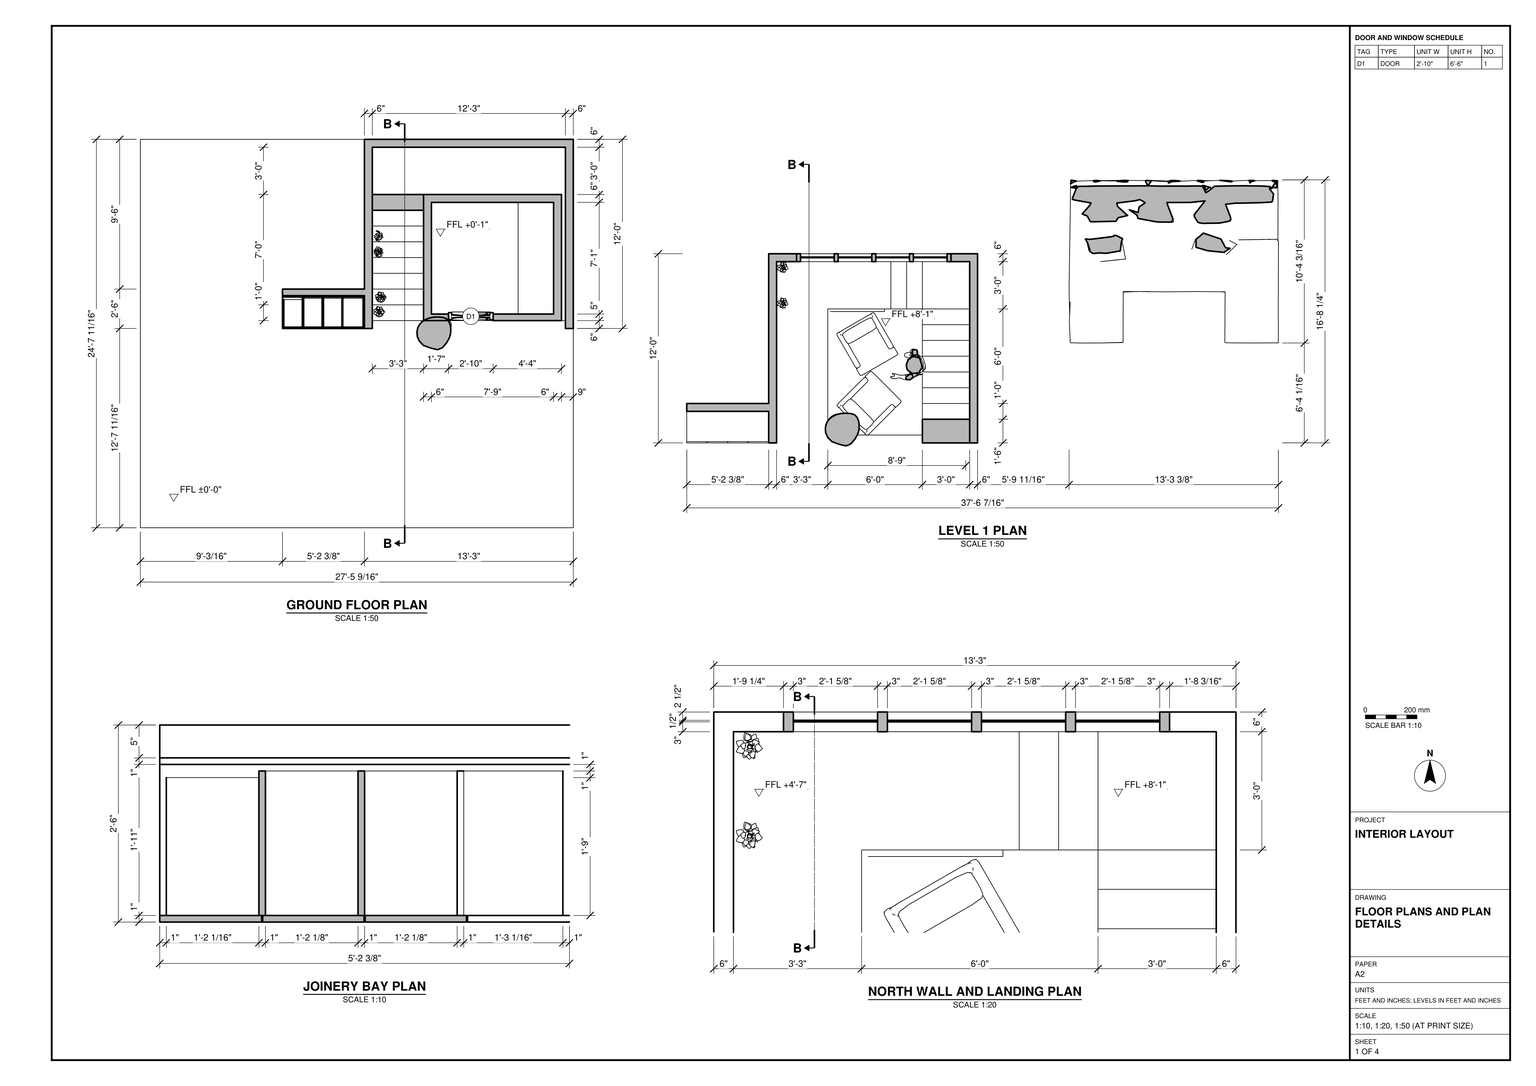
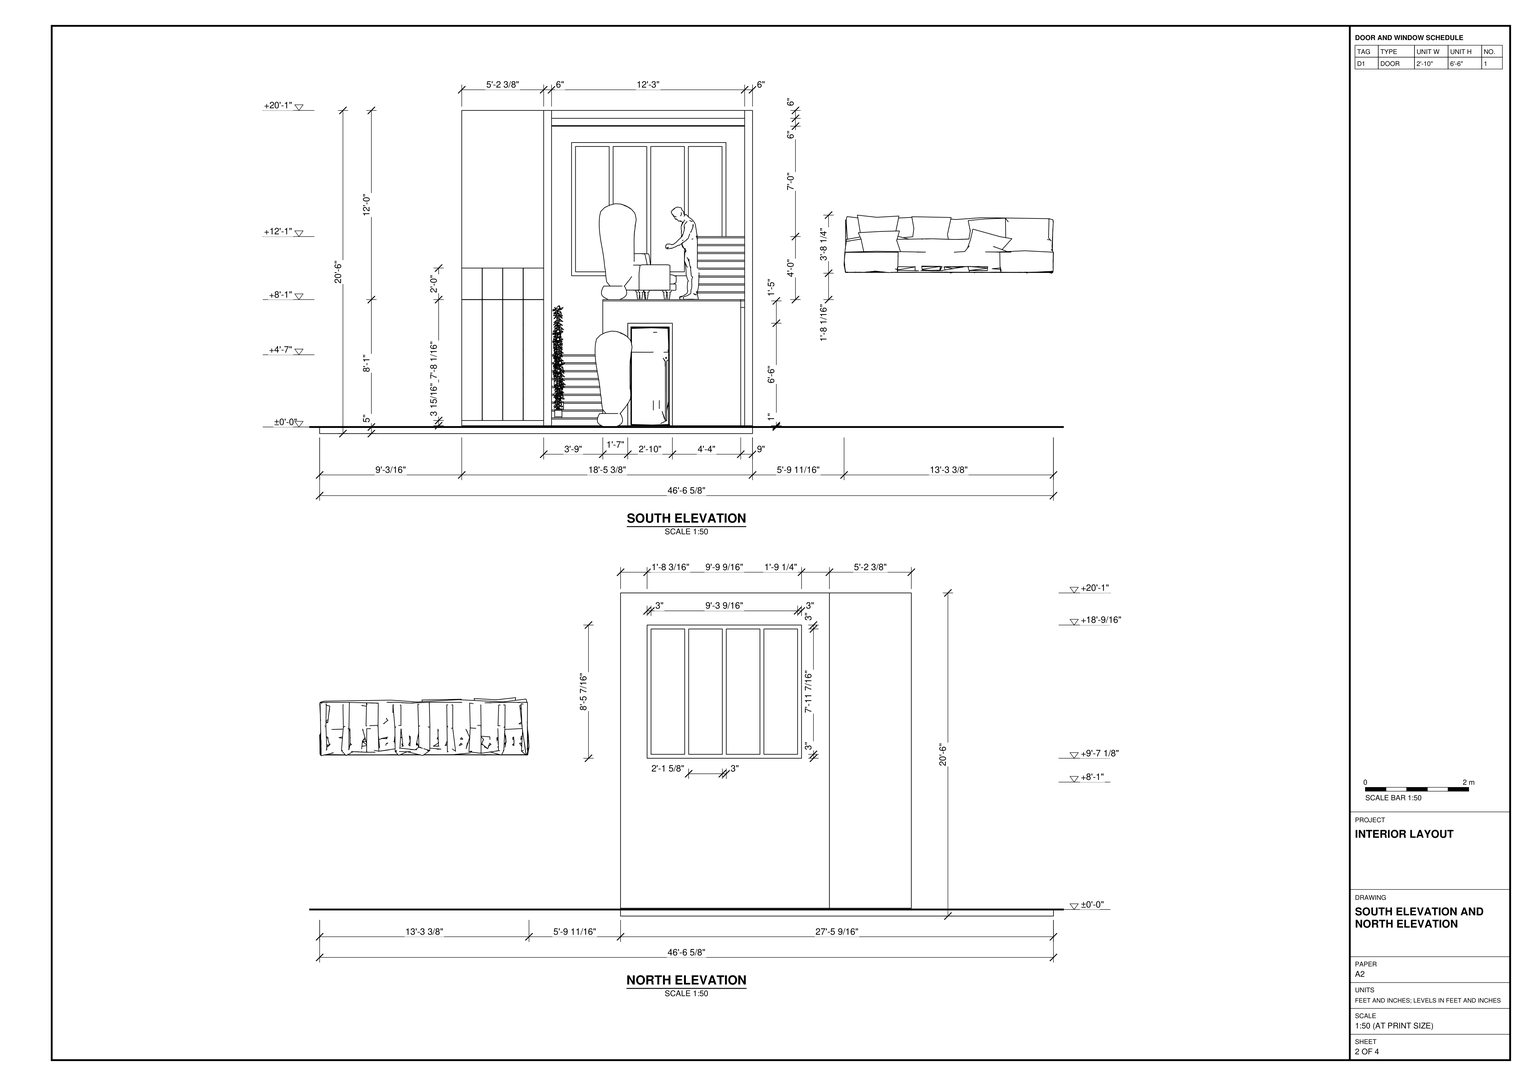
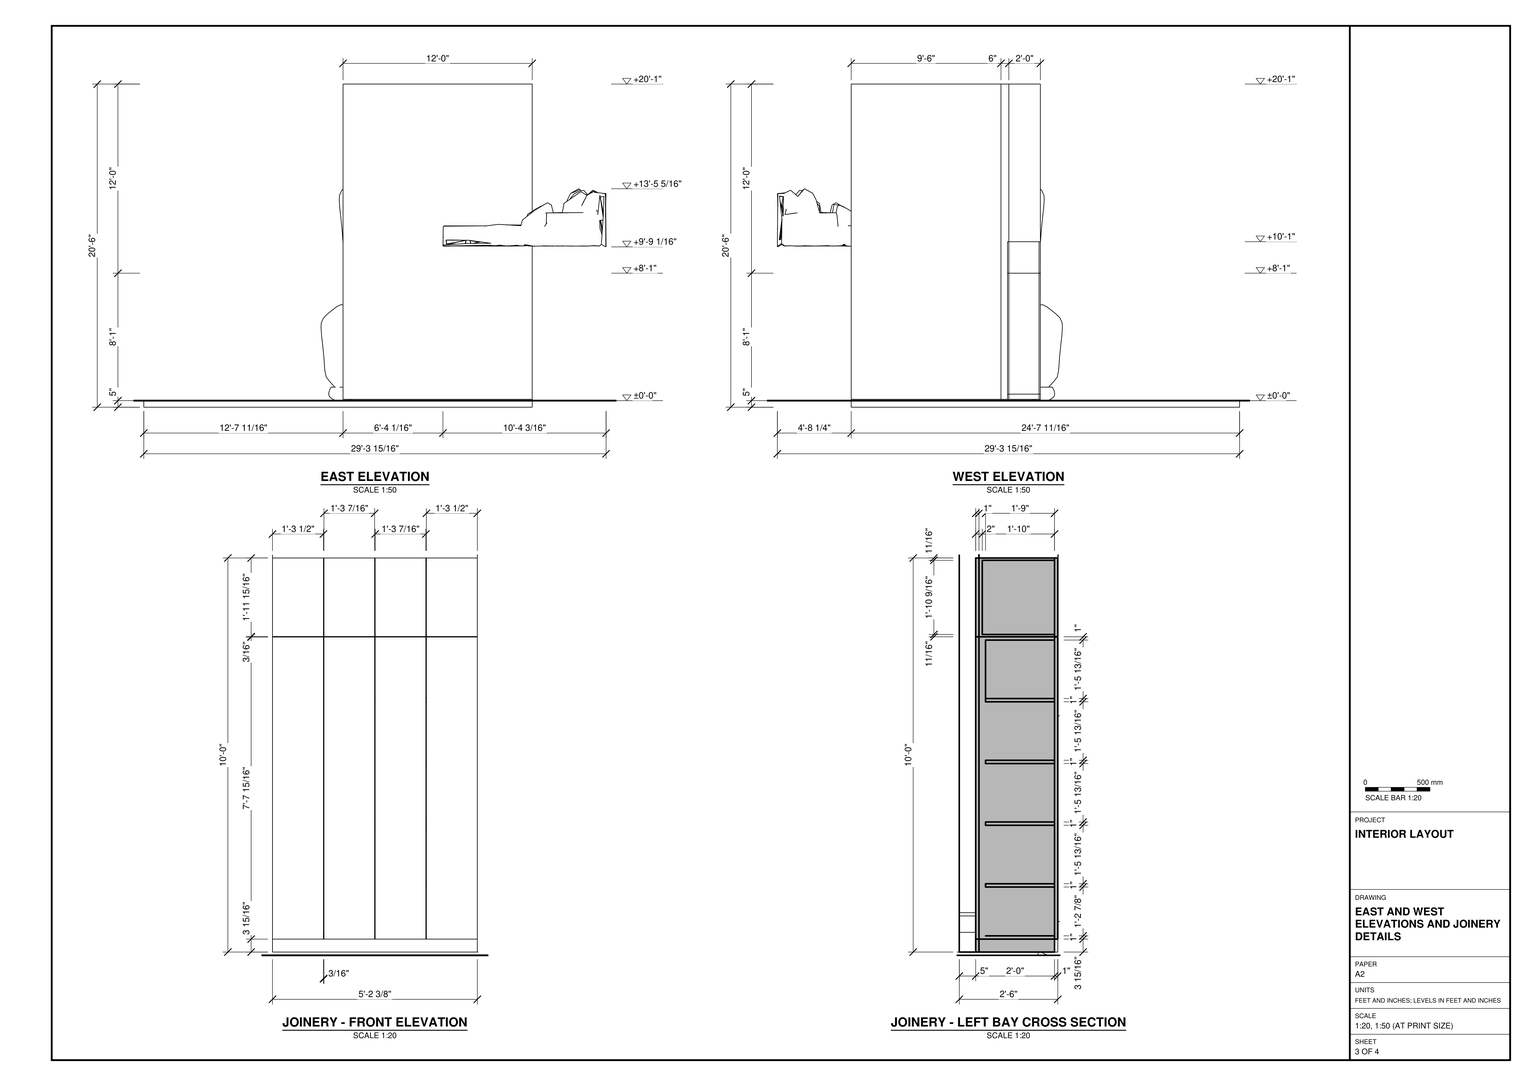
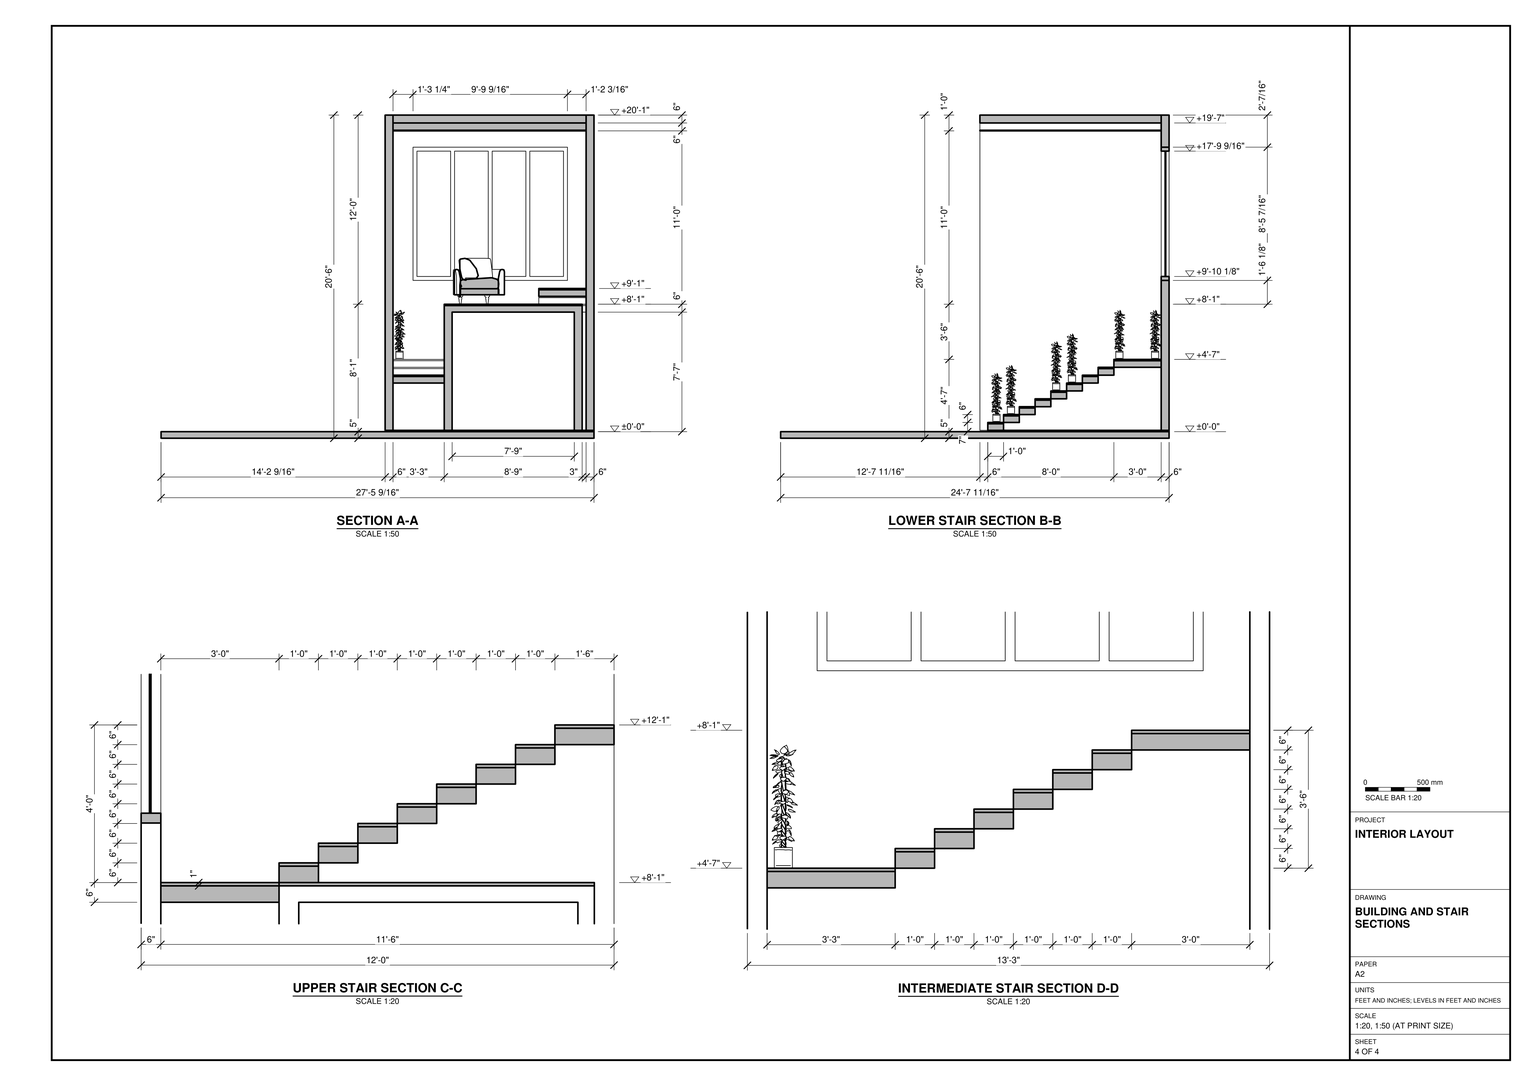
Build the interior in SketchUp from task_files/diagram_01.pdf. Work in feet and inches. The complete layout, including the sofa set apart from the room, measures 46'-6 5/8" east to west, 29'-3 15/16" north to south and 20'-6" high. Set the ground floor at ±0'-0" and the upper floor at +8'-1".

Model the rectangular base slab and place the room and adjacent storage unit in its northeast portion as shown in plan. Build the outer walls, lower room enclosure, upper floor and flat top of the shell, following the wall and slab thicknesses in the drawings. Fit the door beneath the upper seating area and the tall, four-part window in the north wall. Form the stair treads and landings, following the changes in direction from the lower flight beside the room to the upper seating level. Include the stepped run along the east side.

Detail the storage unit to the west of the room using the joinery plan, front elevation and left bay section. Place the two angled chairs on the upper floor. Match the separate sofa's footprint, offset and elevation rather than placing it inside the room. Decor and loose items such as plants, lights and cushions may be any suitable library components. Keep shell elements and individual furniture and joinery pieces in separate groups or components, and use components for repeated parts. Save one SketchUp model as output_files/two_level_interior_with_stairs_seating_and_storage.skp.

# SketchUp Ruby script. Lengths in inches.
U = 1.inch
M = Sketchup.active_model
def pt(a) = Geom::Point3d.new(a.map { |v| v * U })
def face(e, loops, mat)
  f = e.add_face(loops[0].map { |a| pt(a) })
  loops[1..].each { |l| e.add_face(l.map { |a| pt(a) }).erase! }
  f.material = f.back_material = mat if mat
  f
end
# faces: each face lists its corners as indices into pts; further lists are holes
def faces(e, pts, list, mat = nil) = list.each { |f| face(e, (f[0].is_a?(Array) ? f : [f]).map { |l| l.map { |i| pts[i] } }, mat) }
# xy, xz, yz: faces in a plane at the given z, y or x. An outline is a flat list of corners, or four numbers for a rectangle; further outlines are holes
def ring(l) = l.size == 4 ? [[l[0], l[1]], [l[2], l[1]], [l[2], l[3]], [l[0], l[3]]] : l.each_slice(2).to_a
def flat(e, list, mat, &to3) = list.each { |f| face(e, (f[0].is_a?(Array) ? f : [f]).map { |l| ring(l).map { |u, v| to3.(u, v) } }, mat) }
def xy(e, z, list, mat = nil) = flat(e, list, mat) { |x, y| [x, y, z] }
def xz(e, y, list, mat = nil) = flat(e, list, mat) { |x, z| [x, y, z] }
def yz(e, x, list, mat = nil) = flat(e, list, mat) { |y, z| [x, y, z] }
def lines(e, pts, list) = list.each { |a, b| e.add_line(pt(pts[a]), pt(pts[b])) }
# prism: a flat outline (further loops are holes) pulled along v
def prism(e, loops, v, mat = nil)
  f = face(e, loops, mat); d = Geom::Vector3d.new(v.map { |x| x * U })
  f.pushpull(f.normal.samedirection?(d) ? d.length : -d.length)
end
def box(e, o, s, mat = nil) = prism(e, [[o, [o[0] + s[0], o[1], o[2]], [o[0] + s[0], o[1] + s[1], o[2]], [o[0], o[1] + s[1], o[2]]]], [0, 0, s[2]], mat)
def at(x, y, z, deg = 0) = Geom::Transformation.translation(pt([x, y, z])) * Geom::Transformation.rotation(ORIGIN, Z_AXIS, deg.degrees)
def axes(o, x, y, z) = Geom::Transformation.new([*x, 0, *y, 0, *z, 0, *pt(o).to_a, 1])
def part(name) = M.definitions.add(name)
# library, detail: a bought-in or finely detailed component or shape, given as its bounding box
def library(name, o, s) = part(name).tap { |d| box(d.entities, o, s) }
def detail(e, o, s) = box(e.add_group.entities, o, s)
def put(e, d, t, mat = nil) = e.add_instance(d, t).tap { |i| i.material = mat if mat }
def group(e, t, mat = nil) = e.add_group.tap { |g| g.transformation = t; g.material = mat if mat }.entities
root = M.entities
M.materials.add("Flourish Wallpaper in Birch (ZHIFWT)").color = [240, 240, 239]
M.materials.add("Generic").color = [250, 241, 217]
M.materials.add("Granite (YU40S8)").color = [194, 194, 192]
M.materials.add("Oak (WT2QPN)").color = [152, 110, 65]
M.materials.add("clr gls").color = [0, 0, 0]
M.materials["clr gls"].alpha = 0.1
M.materials.add("finishes").color = [136, 230, 240]
c1 = library("Door 243 024",[-21.4,-3.3125,0],[42.8,6.625,82.43])
c2 = library("Europallet Sofa 187 023",[-79.48,-61.95,-1.08],[159.38,124.19,44.26])
c3 = library("Crowd Pleaser Chair",[-16.54,-18.77,0],[33.13,37.25,34.98])
c4 = library("Dome Light",[-12,-12,0],[24,24,12])
c5 = library("Monstera adansonii 006",[-11.3125,-15.55,-0.02],[28.16,28.64,72.98])
c6 = library("Bradley 001 Standing",[-14.36,-9.95,0.01],[28.64,19.87,70.39])
c7 = library("Tall Climbing Plant 50-13",[-4.09,-3.9375,0],[8.41,8.24,37.49])
c8 = part("Group\#13")
box(c8.entities,[0,0,0],[36,12,5])
c9 = part("Group\#23")
box(c9.entities,[0,0,0],[36,12,1])
c10 = library("Group\#21",[0,0,0],[147,138,0.47])
put(root,c1,axes([251.5625,161,0],[0.79447,0,0],[0,1,0],[0,0,0.9463]))
put(root,c2,at(478.74,289.6875,117.13))
put(root,c3,at(245.43,227.05,96,30))
put(root,c3,at(246.87,181.66,96,135))
put(root,c4,at(36.87,157.6875,185))
put(root,c5,at(224.14,164.3,96))
put(root,c5,at(221,150.45,-1))
put(root,c6,at(278.59,208.28,96,-124.262))
put(root,c7,at(181.72,164.28,6))
put(root,c7,at(182.9,175.33,12))
put(root,c7,at(181.38,209.77,30))
put(root,c7,at(181.39,221.77,36))
put(root,c7,at(181.48,257.88,54))
put(root,c7,at(181.51,285.08,54))
put(root,c8,axes([176.5625,157.6875,0],[1.08333,0,0],[0,1,0],[0,0,1]))
g1 = group(root,at(176.5625,157.6875,5),"Granite (YU40S8)")
box(g1,[0,0,0],[39,12,1])
put(root,c9,axes([176.5625,169.6875,11],[1.08333,0,0],[0,1,0],[0,0,1]),"Granite (YU40S8)")
put(root,c8,axes([176.5625,169.6875,6],[1.08333,0,0],[0,1,0],[0,0,1]))
put(root,c9,axes([176.5625,181.6875,17],[1.08333,0,0],[0,1,0],[0,0,1]),"Granite (YU40S8)")
put(root,c8,axes([176.5625,181.6875,12],[1.08333,0,0],[0,1,0],[0,0,1]))
put(root,c9,axes([176.5625,193.6875,23],[1.08333,0,0],[0,1,0],[0,0,1]),"Granite (YU40S8)")
put(root,c8,axes([176.5625,193.6875,18],[1.08333,0,0],[0,1,0],[0,0,1]))
put(root,c9,axes([176.5625,205.6875,29],[1.08333,0,0],[0,1,0],[0,0,1]),"Granite (YU40S8)")
put(root,c8,axes([176.5625,205.6875,24],[1.08333,0,0],[0,1,0],[0,0,1]))
put(root,c9,axes([176.5625,217.6875,35],[1.08333,0,0],[0,1,0],[0,0,1]),"Granite (YU40S8)")
put(root,c8,axes([176.5625,217.6875,30],[1.08333,0,0],[0,1,0],[0,0,1]))
put(root,c9,axes([176.5625,229.6875,41],[1.08333,0,0],[0,1,0],[0,0,1]),"Granite (YU40S8)")
put(root,c8,axes([176.5625,229.6875,36],[1.08333,0,0],[0,1,0],[0,0,1]))
put(root,c9,axes([176.5625,241.6875,47],[1.08333,0,0],[0,1,0],[0,0,1]),"Granite (YU40S8)")
put(root,c8,axes([176.5625,241.6875,42],[1.08333,0,0],[0,1,0],[0,0,1]))
g2 = group(root,at(176.5625,253.6875,53),"Granite (YU40S8)")
box(g2,[0,0,0],[39,36,1])
g3 = group(root,at(176.5625,253.6875,48))
box(g3,[0,0,0],[39,36,5])
put(root,c8,at(227.5625,253.6875,54,90))
put(root,c9,at(227.5625,253.6875,59,90),"Granite (YU40S8)")
put(root,c9,at(287.5625,253.6875,89,90),"Granite (YU40S8)")
put(root,c8,at(287.5625,253.6875,84,90))
g4 = group(root,at(299.5625,253.6875,95,90),"Granite (YU40S8)")
box(g4,[0,-24,0],[36,36,1])
g5 = group(root,at(299.5625,253.6875,90,90))
box(g5,[0,-24,0],[36,36,5])
put(root,c8,at(287.5625,241.6875,96))
put(root,c9,at(287.5625,241.6875,101),"Granite (YU40S8)")
put(root,c8,at(287.5625,229.6875,102))
put(root,c9,at(287.5625,229.6875,107),"Granite (YU40S8)")
put(root,c8,at(287.5625,217.6875,108))
put(root,c9,at(287.5625,217.6875,113),"Granite (YU40S8)")
put(root,c8,at(287.5625,205.6875,114))
put(root,c9,at(287.5625,205.6875,119),"Granite (YU40S8)")
put(root,c8,at(287.5625,193.6875,120))
put(root,c9,at(287.5625,193.6875,125),"Granite (YU40S8)")
put(root,c8,at(287.5625,181.6875,126))
put(root,c9,at(287.5625,181.6875,131),"Granite (YU40S8)")
put(root,c8,at(287.5625,169.6875,132))
put(root,c9,at(287.5625,169.6875,137),"Granite (YU40S8)")
g6 = group(root,at(287.5625,157.6875,138))
box(g6,[0,-6,0],[36,18,5])
g7 = group(root,at(287.5625,157.6875,143),"Granite (YU40S8)")
box(g7,[0,-6,0],[36,18,1])
g8 = group(root,at(173.5625,151.6875,0),"Generic")
xy(g8,0,[[-3,0,-3,24,-65.375,24,-65.375,30,-3,30,-3,144,3,144,3,0],[150,0,150,138,3,138,3,144,156,144,156,0]])
xy(g8,114.13,[[18.23,138,135.79,144]])
xy(g8,215.57,[[18.23,138,135.79,144]])
xy(g8,240,[[-3,0,3,0,3,138,150,138,150,0,156,0,156,144,-3,144,-3,30,-65.375,30,-65.375,24,-3,24]])
xz(g8,0,[[-3,0,3,240],[150,0,156,240]])
xz(g8,24,[[-65.375,0,-3,120],[-65.375,120,-3,240]])
xz(g8,30,[[-65.375,0,-3,240]])
xz(g8,138,[[[3,0,150,240],[18.23,114.13,135.79,215.57]]],"Flourish Wallpaper in Birch (ZHIFWT)")
xz(g8,144,[[[-3,0,156,240],[18.23,114.13,135.79,215.57]]])
yz(g8,-65.375,[[24,0,30,240]])
yz(g8,-3,[[0,0,24,120],[30,0,144,240],[0,120,24,240]])
yz(g8,3,[[0,0,138,240]],"Flourish Wallpaper in Birch (ZHIFWT)")
yz(g8,18.23,[[138,114.13,144,215.57]])
yz(g8,135.79,[[138,114.13,144,215.57]])
yz(g8,150,[[0,0,138,240]],"Flourish Wallpaper in Birch (ZHIFWT)")
yz(g8,156,[[0,0,144,240]])
p = [[42,6,0],[42,102,0],[114,102,0],[114,6,0]]
lines(g8,p,[[0,1],[1,2],[2,3]])
g9 = group(root,at(215.5625,157.6875,0),"Generic")
xy(g9,0,[[0,0,0,96,105,96,105,0,53,0,53,5,99,5,99,90,6,90,6,5,19,5,19,0]])
xy(g9,78,[[19,0,53,5]])
xy(g9,90,[[6,5,99,90]])
xy(g9,95,[[0,0,105,96]])
xz(g9,0,[[0,0,19,0,19,78,53,78,53,0,105,0,105,95,0,95]])
xz(g9,5,[[6,0,19,90],[53,0,99,90],[19,78,53,90]])
xz(g9,90,[[6,0,99,90]])
xz(g9,96,[[0,0,105,95]])
yz(g9,0,[[0,0,96,95]])
yz(g9,6,[[5,0,90,90]])
yz(g9,19,[[0,0,5,78]])
yz(g9,53,[[0,0,5,78]])
yz(g9,99,[[5,0,90,90]])
yz(g9,105,[[0,0,96,95]])
p = [[19,0,90],[19,5,90],[53,0,90],[53,5,90],[43.05,94,96],[2,94,96],
  [43.05,96,96]]
lines(g9,p,[[0,1],[2,3],[4,5],[4,6]])
g10 = group(root,at(221.5625,157.6875,-1))
box(g10,[-45,0,0],[153,138,1])
g11 = group(root,at(221.5625,157.6875,-6))
box(g11,[-221.5625,-157.6875,0],[329.5625,295.6875,5])
g12 = group(root,at(108.1875,152.6875,0),"finishes")
xy(g12,3.9375,[[0,0,62.375,24]])
xy(g12,4.9375,[[1,0,15.09,21],[15.09,0,16.09,22],[16.09,0,30.1875,22],[30.1875,0,31.1875,22],[31.1875,0,45.28,22],
  [45.28,0,61.375,22]])
xy(g12,19.8,[[1,0,15.09,21],[46.28,0,61.375,22]])
xy(g12,20.8,[[1,0,15.09,21],[46.28,0,61.375,22]])
xy(g12,38.6,[[1,0,15.09,21],[16.09,0,30.1875,22],[31.1875,0,45.28,22],[46.28,0,61.375,22]])
xy(g12,39.6,[[1,0,15.09,21],[16.09,0,30.1875,22],[31.1875,0,45.28,22],[46.28,0,61.375,22]])
xy(g12,57.4,[[1,0,15.09,21],[46.28,0,61.375,22]])
xy(g12,58.4,[[1,0,15.09,21],[46.28,0,61.375,22]])
xy(g12,76.2,[[1,0,15.09,21],[16.09,0,30.1875,22],[31.1875,0,45.28,22],[46.28,0,61.375,22]])
xy(g12,77.2,[[1,0,15.09,21],[16.09,0,30.1875,22],[31.1875,0,45.28,22],[46.28,0,61.375,22]])
xy(g12,95,[[1,0,15.09,21],[16.09,0,30.1875,22],[31.1875,0,45.28,22],[46.28,0,61.375,22]])
xy(g12,96,[[0,0,62.375,24]])
xz(g12,0,[[[0,3.9375,62.375,96],[1,4.9375,1,19.8,15.09,19.8,15.09,4.9375,16.09,4.9375,16.09,95,30.1875,95,30.1875,77.2,16.09,77.2,16.09,76.2,30.1875,76.2,30.1875,39.6,16.09,39.6,16.09,38.6,30.1875,38.6,30.1875,4.9375,31.1875,4.9375,31.1875,95,45.28,95,45.28,77.2,31.1875,77.2,31.1875,76.2,45.28,76.2,45.28,39.6,31.1875,39.6,31.1875,38.6,45.28,38.6,45.28,4.9375,46.28,4.9375,46.28,95,61.375,95,61.375,77.2,46.28,77.2,46.28,76.2,61.375,76.2,61.375,58.4,46.28,58.4,46.28,57.4,61.375,57.4,61.375,39.6,46.28,39.6,46.28,38.6,61.375,38.6,61.375,20.8,46.28,20.8,46.28,19.8,61.375,19.8,61.375,4.9375],[1,39.6,15.09,57.4],[1,20.8,15.09,38.6],[1,77.2,15.09,95],[1,58.4,15.09,76.2]]])
xz(g12,21,[[1,19.8,15.09,20.8],[1,38.6,15.09,39.6],[1,57.4,15.09,58.4],[1,76.2,15.09,77.2],[1,77.2,15.09,95]])
xz(g12,22,[[15.09,4.9375,16.09,95],[30.1875,4.9375,31.1875,4.9375,31.1875,95,30.1875,95,30.1875,77.2,16.09,77.2,16.09,76.2,30.1875,76.2,30.1875,39.6,16.09,39.6,16.09,38.6,30.1875,38.6],[45.28,4.9375,46.28,4.9375,46.28,95,45.28,95,45.28,77.2,31.1875,77.2,31.1875,76.2,45.28,76.2,45.28,39.6,31.1875,39.6,31.1875,38.6,45.28,38.6],[46.28,19.8,61.375,20.8],[46.28,38.6,61.375,39.6],
  [46.28,57.4,61.375,58.4],[46.28,76.2,61.375,77.2],[16.09,77.2,30.1875,95],[31.1875,77.2,45.28,95],[46.28,77.2,61.375,95]])
xz(g12,24,[[0,3.9375,62.375,96]])
yz(g12,0,[[0,3.9375,24,96]])
yz(g12,1,[[0,4.9375,21,19.8],[0,20.8,21,38.6],[0,39.6,21,57.4],[0,58.4,21,76.2],[0,77.2,21,95]])
yz(g12,15.09,[[0,4.9375,0,19.8,21,19.8,21,20.8,0,20.8,0,38.6,21,38.6,21,39.6,0,39.6,0,57.4,21,57.4,21,58.4,0,58.4,0,76.2,21,76.2,21,95,22,95,22,4.9375],[0,77.2,21,95]])
yz(g12,16.09,[[0,4.9375,22,19.8],[0,38.6,22,39.6],[0,39.6,22,57.4],[0,76.2,22,77.2],[0,77.2,22,95]])
yz(g12,30.1875,[[0,4.9375,22,38.6],[0,39.6,22,76.2],[0,77.2,22,95]])
yz(g12,31.1875,[[0,4.9375,22,19.8],[0,38.6,22,39.6],[0,39.6,22,57.4],[0,76.2,22,77.2],[0,77.2,22,95]])
yz(g12,45.28,[[0,4.9375,22,38.6],[0,39.6,22,76.2],[0,77.2,22,95]])
yz(g12,46.28,[[0,19.8,22,20.8],[0,38.6,22,39.6],[0,57.4,22,58.4],[0,76.2,22,77.2],[0,77.2,22,95]])
yz(g12,61.375,[[0,4.9375,22,19.8],[0,20.8,22,38.6],[0,39.6,22,57.4],[0,58.4,22,76.2],[0,77.2,22,95]])
yz(g12,62.375,[[0,3.9375,24,96]])
g13 = group(root,at(108.1875,151.6875,0),"finishes")
box(g13,[0,0,3.9375],[15.52,1,91.98])
box(g13,[15.67,0,3.9375],[15.44,1,91.98])
box(g13,[31.27,0,3.9375],[15.43,1,91.98])
box(g13,[46.86,0,3.9375],[15.52,1,91.98])
box(g13,[46.86,0,96.08],[15.52,1,23.92])
box(g13,[31.27,0,96.08],[15.43,1,23.92])
box(g13,[15.67,0,96.08],[15.44,1,23.92])
box(g13,[0,0,96.08],[15.52,1,23.92])
g14 = group(root,at(108.1875,152.6875,96),"finishes")
xy(g14,0,[[0,0,62.375,24]])
xy(g14,0.71,[[0.71,0,14.95,22],[14.95,0,15.95,22],[30.1875,0,31.1875,22],[45.43,0,46.43,22]])
xy(g14,23.29,[[0.71,0,14.95,22],[15.95,0,30.1875,22],[31.1875,0,45.43,22],[46.43,0,61.67,22]])
xy(g14,24,[[0,0,62.375,24]])
xz(g14,0,[[[0,0,62.375,24],[0.71,0.71,0.71,23.29,14.95,23.29,14.95,0.71,15.95,0.71,15.95,23.29,30.1875,23.29,30.1875,0.71,31.1875,0.71,31.1875,23.29,45.43,23.29,45.43,0.71,46.43,0.71,46.43,23.29,61.67,23.29,61.67,0.71]]])
xz(g14,22,[[0.71,0.71,14.95,23.29],[14.95,0.71,15.95,23.29],[30.1875,0.71,31.1875,23.29],[45.43,0.71,46.43,23.29]])
xz(g14,24,[[0,0,62.375,24]])
yz(g14,0,[[0,0,24,24]])
yz(g14,0.71,[[0,0.71,22,23.29]])
yz(g14,14.95,[[0,0.71,22,23.29]])
yz(g14,15.95,[[0,0.71,22,23.29]])
yz(g14,30.1875,[[0,0.71,22,23.29]])
yz(g14,31.1875,[[0,0.71,22,23.29]])
yz(g14,45.43,[[0,0.71,22,23.29]])
yz(g14,46.43,[[0,0.71,22,23.29]])
yz(g14,61.67,[[0,0.71,22,23.29]])
yz(g14,62.375,[[0,0,24,24]])
g15 = group(root,at(108.1875,151.6875,0))
box(g15,[0,1,0],[62.375,24,3.9375])
g16 = group(root,at(191.79,289.6875,114.13),"Oak (WT2QPN)")
prism(g16,[[[117.5625,0,0],[117.5625,0,101.4375],[0,0,101.4375],[0,0,98.4375],[0,0,3],[0,0,0]],[[88.92,0,3],[88.92,0,98.4375],[114.5625,0,98.4375],[114.5625,0,3]],[[60.28,0,3],[60.28,0,98.4375],[85.92,0,98.4375],[85.92,0,3]],[[31.64,0,3],[31.64,0,98.4375],[57.28,0,98.4375],[57.28,0,3]],[[3,0,3],[3,0,98.4375],[28.64,0,98.4375],[28.64,0,3]]],[0,6,0])
g17 = group(root,at(194.79,292.6875,117.13),"clr gls")
box(g17,[28.64,0,0],[25.64,0.47,95.4375])
box(g17,[57.28,0,0],[25.64,0.47,95.4375])
box(g17,[85.92,0,0],[25.64,0.47,95.4375])
box(g17,[0,0,0],[25.64,0.47,95.4375])
put(root,c10,axes([176.5625,151.6875,228.47],[1,0,0],[0,1,0],[0,0,-1]))
g18 = group(root,at(176.5625,151.6875,234))
box(g18,[0,0,0],[147,138,6])
put(root,c9,at(275.5625,253.6875,83,90),"Granite (YU40S8)")
put(root,c8,at(275.5625,253.6875,78,90))
put(root,c9,at(263.5625,253.6875,77,90),"Granite (YU40S8)")
put(root,c8,at(263.5625,253.6875,72,90))
put(root,c9,at(251.5625,253.6875,71,90),"Granite (YU40S8)")
put(root,c8,at(251.5625,253.6875,66,90))
put(root,c9,at(239.5625,253.6875,65,90),"Granite (YU40S8)")
put(root,c8,at(239.5625,253.6875,60,90))
g19 = group(root,at(215.5625,157.6875,95),"Granite (YU40S8)")
box(g19,[0,0,0],[105,96,1])
